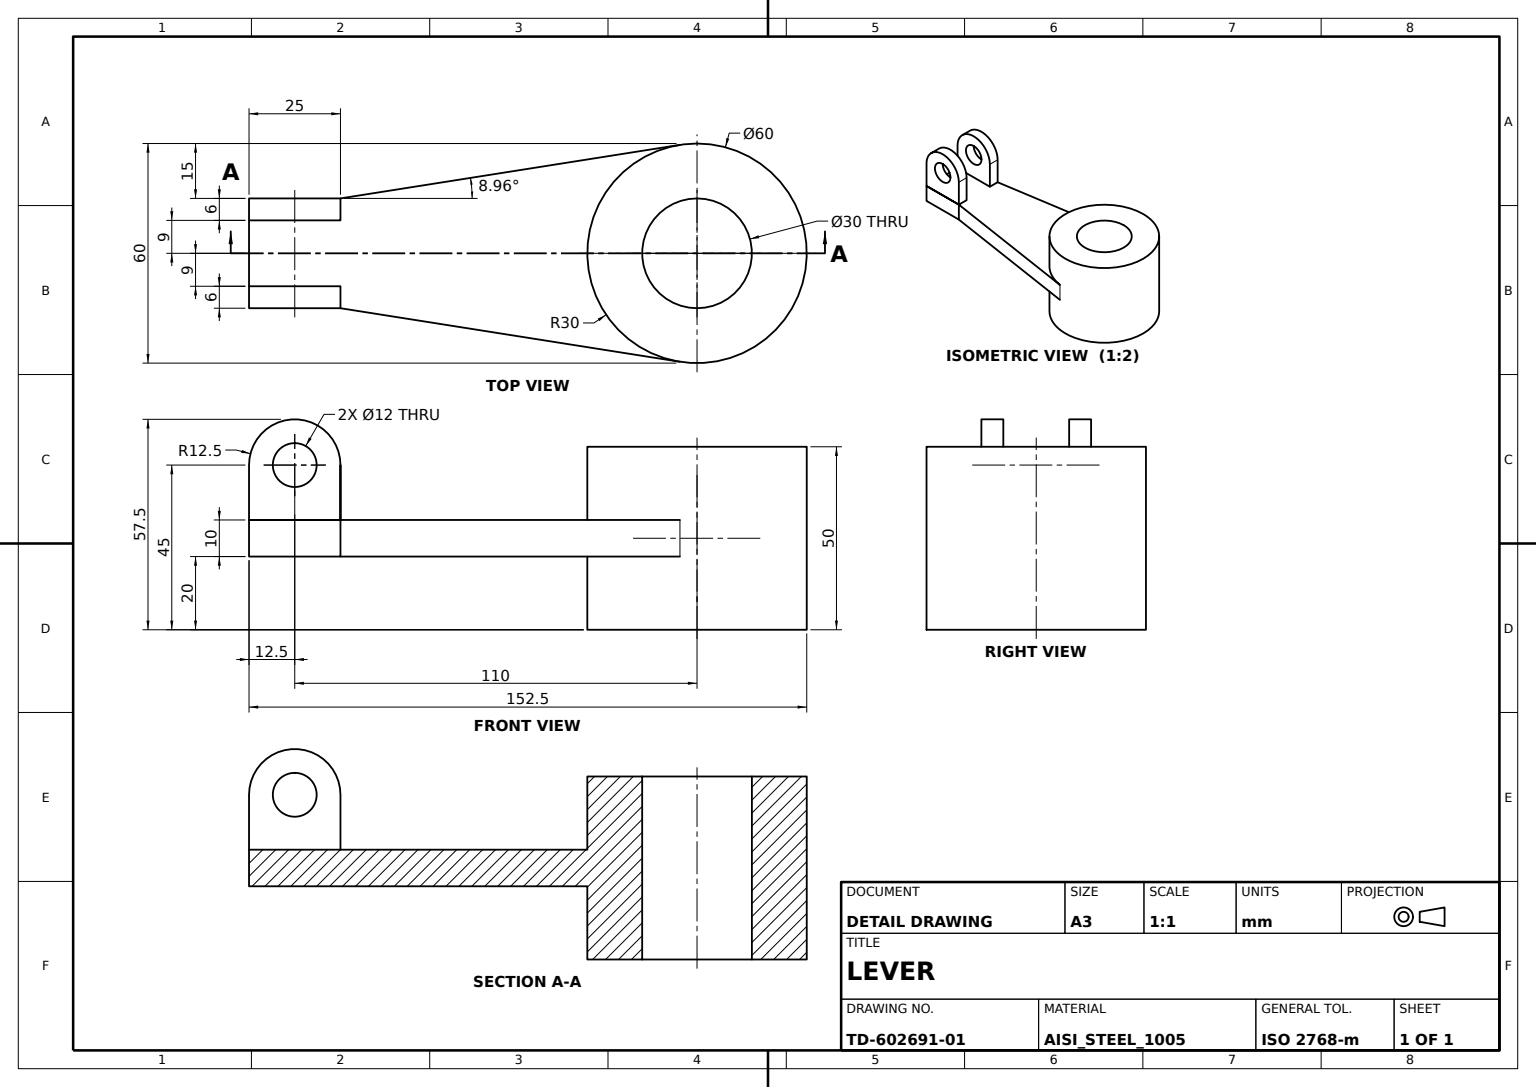
ISO-10303-21;
HEADER;
FILE_DESCRIPTION((''),'2;1');
FILE_NAME('','',(''),(''),'','','');
FILE_SCHEMA(('AUTOMOTIVE_DESIGN'));
ENDSEC;
DATA;
#1=APPLICATION_CONTEXT('');
#2=PRODUCT_CONTEXT('',#1,'mechanical');
#3=PRODUCT('','','',(#2));
#4=PRODUCT_DEFINITION_FORMATION('','',#3);
#5=PRODUCT_DEFINITION_CONTEXT('',#1,'design');
#6=PRODUCT_DEFINITION('','',#4,#5);
#7=PRODUCT_DEFINITION_SHAPE('','',#6);
#8=(LENGTH_UNIT()NAMED_UNIT(*)SI_UNIT(.MILLI.,.METRE.));
#9=(NAMED_UNIT(*)PLANE_ANGLE_UNIT()SI_UNIT($,.RADIAN.));
#10=(NAMED_UNIT(*)SI_UNIT($,.STERADIAN.)SOLID_ANGLE_UNIT());
#11=UNCERTAINTY_MEASURE_WITH_UNIT(LENGTH_MEASURE(0.005),#8,'distance_accuracy_value','');
#12=(GEOMETRIC_REPRESENTATION_CONTEXT(3)GLOBAL_UNCERTAINTY_ASSIGNED_CONTEXT((#11))GLOBAL_UNIT_ASSIGNED_CONTEXT((#8,#9,#10))REPRESENTATION_CONTEXT('',''));
#13=CARTESIAN_POINT('',(-122.5,9.,5.));
#14=VERTEX_POINT('',#13);
#15=CARTESIAN_POINT('',(-122.5,15.,5.));
#16=VERTEX_POINT('',#15);
#17=DIRECTION('',(0.,1.,0.));
#18=VECTOR('',#17,1000.);
#19=LINE('',#13,#18);
#20=EDGE_CURVE('',#14,#16,#19,.T.);
#21=ORIENTED_EDGE('',*,*,#20,.F.);
#22=CARTESIAN_POINT('',(-122.5,9.,20.));
#23=VERTEX_POINT('',#22);
#24=DIRECTION('',(0.,0.,-1.));
#25=VECTOR('',#24,1000.);
#26=LINE('',#22,#25);
#27=EDGE_CURVE('',#23,#14,#26,.T.);
#28=ORIENTED_EDGE('',*,*,#27,.F.);
#29=CARTESIAN_POINT('',(-122.5,15.,20.));
#30=VERTEX_POINT('',#29);
#31=LINE('',#22,#18);
#32=EDGE_CURVE('',#23,#30,#31,.T.);
#33=ORIENTED_EDGE('',*,*,#32,.T.);
#34=LINE('',#29,#25);
#35=EDGE_CURVE('',#30,#16,#34,.T.);
#36=ORIENTED_EDGE('',*,*,#35,.T.);
#37=EDGE_LOOP('',(#21,#28,#33,#36));
#38=FACE_BOUND('',#37,.T.);
#39=DIRECTION('',(1.,0.,0.));
#40=AXIS2_PLACEMENT_3D('',#22,#39,#17);
#41=PLANE('',#40);
#42=ADVANCED_FACE('',(#38),#41,.F.);
#43=CARTESIAN_POINT('',(-110.,9.,26.));
#44=VERTEX_POINT('',#43);
#45=CARTESIAN_POINT('',(-110.,9.,20.));
#46=DIRECTION('',(0.,-1.,0.));
#47=DIRECTION('',(0.,0.,1.));
#48=AXIS2_PLACEMENT_3D('',#45,#46,#47);
#49=CIRCLE('',#48,6.);
#50=EDGE_CURVE('',#44,#44,#49,.T.);
#51=ORIENTED_EDGE('',*,*,#50,.T.);
#52=EDGE_LOOP('',(#51));
#53=FACE_BOUND('',#52,.T.);
#54=CARTESIAN_POINT('',(-110.,15.,26.));
#55=VERTEX_POINT('',#54);
#56=CARTESIAN_POINT('',(-110.,15.,20.));
#57=AXIS2_PLACEMENT_3D('',#56,#46,#47);
#58=CIRCLE('',#57,6.);
#59=EDGE_CURVE('',#55,#55,#58,.T.);
#60=ORIENTED_EDGE('',*,*,#59,.F.);
#61=EDGE_LOOP('',(#60));
#62=FACE_BOUND('',#61,.T.);
#63=DIRECTION('',(-1.,0.,0.));
#64=AXIS2_PLACEMENT_3D('',#45,#17,#63);
#65=CYLINDRICAL_SURFACE('',#64,6.);
#66=ADVANCED_FACE('',(#53,#62),#65,.F.);
#67=CARTESIAN_POINT('',(-97.5,9.,5.));
#68=VERTEX_POINT('',#67);
#69=CARTESIAN_POINT('',(-97.5,15.,5.));
#70=VERTEX_POINT('',#69);
#71=LINE('',#67,#18);
#72=EDGE_CURVE('',#68,#70,#71,.T.);
#73=ORIENTED_EDGE('',*,*,#72,.F.);
#74=VECTOR('',#39,1000.);
#75=LINE('',#13,#74);
#76=EDGE_CURVE('',#14,#68,#75,.T.);
#77=ORIENTED_EDGE('',*,*,#76,.F.);
#78=ORIENTED_EDGE('',*,*,#20,.T.);
#79=LINE('',#15,#74);
#80=EDGE_CURVE('',#16,#70,#79,.T.);
#81=ORIENTED_EDGE('',*,*,#80,.T.);
#82=EDGE_LOOP('',(#73,#77,#78,#81));
#83=FACE_BOUND('',#82,.T.);
#84=AXIS2_PLACEMENT_3D('',#13,#47,#39);
#85=PLANE('',#84);
#86=ADVANCED_FACE('',(#83),#85,.F.);
#87=ORIENTED_EDGE('',*,*,#32,.F.);
#88=CARTESIAN_POINT('',(-97.5,9.,20.));
#89=VERTEX_POINT('',#88);
#90=CIRCLE('',#48,12.5);
#91=EDGE_CURVE('',#89,#23,#90,.T.);
#92=ORIENTED_EDGE('',*,*,#91,.F.);
#93=CARTESIAN_POINT('',(-97.5,15.,20.));
#94=VERTEX_POINT('',#93);
#95=LINE('',#88,#18);
#96=EDGE_CURVE('',#89,#94,#95,.T.);
#97=ORIENTED_EDGE('',*,*,#96,.T.);
#98=CIRCLE('',#57,12.5);
#99=EDGE_CURVE('',#94,#30,#98,.T.);
#100=ORIENTED_EDGE('',*,*,#99,.T.);
#101=EDGE_LOOP('',(#87,#92,#97,#100));
#102=FACE_BOUND('',#101,.T.);
#103=CYLINDRICAL_SURFACE('',#64,12.5);
#104=ADVANCED_FACE('',(#102),#103,.T.);
#105=ORIENTED_EDGE('',*,*,#96,.F.);
#106=VECTOR('',#47,1000.);
#107=LINE('',#67,#106);
#108=EDGE_CURVE('',#68,#89,#107,.T.);
#109=ORIENTED_EDGE('',*,*,#108,.F.);
#110=ORIENTED_EDGE('',*,*,#72,.T.);
#111=LINE('',#69,#106);
#112=EDGE_CURVE('',#70,#94,#111,.T.);
#113=ORIENTED_EDGE('',*,*,#112,.T.);
#114=EDGE_LOOP('',(#105,#109,#110,#113));
#115=FACE_BOUND('',#114,.T.);
#116=AXIS2_PLACEMENT_3D('',#67,#63,#46);
#117=PLANE('',#116);
#118=ADVANCED_FACE('',(#115),#117,.F.);
#119=ORIENTED_EDGE('',*,*,#59,.T.);
#120=EDGE_LOOP('',(#119));
#121=FACE_BOUND('',#120,.T.);
#122=ORIENTED_EDGE('',*,*,#80,.F.);
#123=ORIENTED_EDGE('',*,*,#35,.F.);
#124=ORIENTED_EDGE('',*,*,#99,.F.);
#125=ORIENTED_EDGE('',*,*,#112,.F.);
#126=EDGE_LOOP('',(#122,#123,#124,#125));
#127=FACE_BOUND('',#126,.T.);
#128=AXIS2_PLACEMENT_3D('',#56,#46,#39);
#129=PLANE('',#128);
#130=ADVANCED_FACE('',(#121,#127),#129,.F.);
#131=ORIENTED_EDGE('',*,*,#108,.T.);
#132=ORIENTED_EDGE('',*,*,#91,.T.);
#133=ORIENTED_EDGE('',*,*,#27,.T.);
#134=ORIENTED_EDGE('',*,*,#76,.T.);
#135=EDGE_LOOP('',(#131,#132,#133,#134));
#136=FACE_BOUND('',#135,.T.);
#137=ORIENTED_EDGE('',*,*,#50,.F.);
#138=EDGE_LOOP('',(#137));
#139=FACE_BOUND('',#138,.T.);
#140=AXIS2_PLACEMENT_3D('',#45,#46,#39);
#141=PLANE('',#140);
#142=ADVANCED_FACE('',(#136,#139),#141,.T.);
#143=CLOSED_SHELL('',(#42,#66,#86,#104,#118,#130,#142));
#144=MANIFOLD_SOLID_BREP('',#143);
#145=CARTESIAN_POINT('',(-122.5,-9.,5.));
#146=VERTEX_POINT('',#145);
#147=CARTESIAN_POINT('',(-97.5,-9.,5.));
#148=VERTEX_POINT('',#147);
#149=LINE('',#145,#74);
#150=EDGE_CURVE('',#146,#148,#149,.T.);
#151=ORIENTED_EDGE('',*,*,#150,.T.);
#152=CARTESIAN_POINT('',(-97.5,-15.,5.));
#153=VERTEX_POINT('',#152);
#154=VECTOR('',#46,1000.);
#155=LINE('',#147,#154);
#156=EDGE_CURVE('',#148,#153,#155,.T.);
#157=ORIENTED_EDGE('',*,*,#156,.T.);
#158=CARTESIAN_POINT('',(-122.5,-15.,5.));
#159=VERTEX_POINT('',#158);
#160=LINE('',#158,#74);
#161=EDGE_CURVE('',#159,#153,#160,.T.);
#162=ORIENTED_EDGE('',*,*,#161,.F.);
#163=LINE('',#145,#154);
#164=EDGE_CURVE('',#146,#159,#163,.T.);
#165=ORIENTED_EDGE('',*,*,#164,.F.);
#166=EDGE_LOOP('',(#151,#157,#162,#165));
#167=FACE_BOUND('',#166,.T.);
#168=AXIS2_PLACEMENT_3D('',#145,#24,#63);
#169=PLANE('',#168);
#170=ADVANCED_FACE('',(#167),#169,.T.);
#171=CARTESIAN_POINT('',(-97.5,-15.,20.));
#172=VERTEX_POINT('',#171);
#173=CARTESIAN_POINT('',(-122.5,-15.,20.));
#174=VERTEX_POINT('',#173);
#175=CARTESIAN_POINT('',(-110.,-15.,20.));
#176=AXIS2_PLACEMENT_3D('',#175,#46,#47);
#177=CIRCLE('',#176,12.5);
#178=EDGE_CURVE('',#172,#174,#177,.T.);
#179=ORIENTED_EDGE('',*,*,#178,.F.);
#180=CARTESIAN_POINT('',(-97.5,-9.,20.));
#181=VERTEX_POINT('',#180);
#182=LINE('',#180,#154);
#183=EDGE_CURVE('',#181,#172,#182,.T.);
#184=ORIENTED_EDGE('',*,*,#183,.F.);
#185=CARTESIAN_POINT('',(-122.5,-9.,20.));
#186=VERTEX_POINT('',#185);
#187=CARTESIAN_POINT('',(-110.,-9.,20.));
#188=AXIS2_PLACEMENT_3D('',#187,#46,#47);
#189=CIRCLE('',#188,12.5);
#190=EDGE_CURVE('',#181,#186,#189,.T.);
#191=ORIENTED_EDGE('',*,*,#190,.T.);
#192=LINE('',#185,#154);
#193=EDGE_CURVE('',#186,#174,#192,.T.);
#194=ORIENTED_EDGE('',*,*,#193,.T.);
#195=EDGE_LOOP('',(#179,#184,#191,#194));
#196=FACE_BOUND('',#195,.T.);
#197=AXIS2_PLACEMENT_3D('',#187,#46,#39);
#198=CYLINDRICAL_SURFACE('',#197,12.5);
#199=ADVANCED_FACE('',(#196),#198,.T.);
#200=CARTESIAN_POINT('',(-110.,-9.,26.));
#201=VERTEX_POINT('',#200);
#202=CIRCLE('',#188,6.);
#203=EDGE_CURVE('',#201,#201,#202,.T.);
#204=ORIENTED_EDGE('',*,*,#203,.F.);
#205=EDGE_LOOP('',(#204));
#206=FACE_BOUND('',#205,.T.);
#207=CARTESIAN_POINT('',(-110.,-15.,26.));
#208=VERTEX_POINT('',#207);
#209=CIRCLE('',#176,6.);
#210=EDGE_CURVE('',#208,#208,#209,.T.);
#211=ORIENTED_EDGE('',*,*,#210,.T.);
#212=EDGE_LOOP('',(#211));
#213=FACE_BOUND('',#212,.T.);
#214=CYLINDRICAL_SURFACE('',#197,6.);
#215=ADVANCED_FACE('',(#206,#213),#214,.F.);
#216=ORIENTED_EDGE('',*,*,#203,.T.);
#217=EDGE_LOOP('',(#216));
#218=FACE_BOUND('',#217,.T.);
#219=ORIENTED_EDGE('',*,*,#190,.F.);
#220=LINE('',#147,#106);
#221=EDGE_CURVE('',#148,#181,#220,.T.);
#222=ORIENTED_EDGE('',*,*,#221,.F.);
#223=ORIENTED_EDGE('',*,*,#150,.F.);
#224=LINE('',#185,#25);
#225=EDGE_CURVE('',#186,#146,#224,.T.);
#226=ORIENTED_EDGE('',*,*,#225,.F.);
#227=EDGE_LOOP('',(#219,#222,#223,#226));
#228=FACE_BOUND('',#227,.T.);
#229=PLANE('',#197);
#230=ADVANCED_FACE('',(#218,#228),#229,.F.);
#231=ORIENTED_EDGE('',*,*,#164,.T.);
#232=LINE('',#173,#25);
#233=EDGE_CURVE('',#174,#159,#232,.T.);
#234=ORIENTED_EDGE('',*,*,#233,.F.);
#235=ORIENTED_EDGE('',*,*,#193,.F.);
#236=ORIENTED_EDGE('',*,*,#225,.T.);
#237=EDGE_LOOP('',(#231,#234,#235,#236));
#238=FACE_BOUND('',#237,.T.);
#239=AXIS2_PLACEMENT_3D('',#185,#63,#46);
#240=PLANE('',#239);
#241=ADVANCED_FACE('',(#238),#240,.T.);
#242=LINE('',#152,#106);
#243=EDGE_CURVE('',#153,#172,#242,.T.);
#244=ORIENTED_EDGE('',*,*,#243,.F.);
#245=ORIENTED_EDGE('',*,*,#156,.F.);
#246=ORIENTED_EDGE('',*,*,#221,.T.);
#247=ORIENTED_EDGE('',*,*,#183,.T.);
#248=EDGE_LOOP('',(#244,#245,#246,#247));
#249=FACE_BOUND('',#248,.T.);
#250=AXIS2_PLACEMENT_3D('',#147,#39,#17);
#251=PLANE('',#250);
#252=ADVANCED_FACE('',(#249),#251,.T.);
#253=ORIENTED_EDGE('',*,*,#210,.F.);
#254=EDGE_LOOP('',(#253));
#255=FACE_BOUND('',#254,.T.);
#256=ORIENTED_EDGE('',*,*,#161,.T.);
#257=ORIENTED_EDGE('',*,*,#243,.T.);
#258=ORIENTED_EDGE('',*,*,#178,.T.);
#259=ORIENTED_EDGE('',*,*,#233,.T.);
#260=EDGE_LOOP('',(#256,#257,#258,#259));
#261=FACE_BOUND('',#260,.T.);
#262=AXIS2_PLACEMENT_3D('',#175,#46,#39);
#263=PLANE('',#262);
#264=ADVANCED_FACE('',(#255,#261),#263,.T.);
#265=CLOSED_SHELL('',(#170,#199,#215,#230,#241,#252,#264));
#266=MANIFOLD_SOLID_BREP('',#265);
#267=VERTEX_POINT('',#15);
#268=VERTEX_POINT('',#158);
#269=LINE('',#15,#154);
#270=EDGE_CURVE('',#267,#268,#269,.T.);
#271=ORIENTED_EDGE('',*,*,#270,.F.);
#272=CARTESIAN_POINT('',(-122.5,15.,-5.));
#273=VERTEX_POINT('',#272);
#274=LINE('',#15,#25);
#275=EDGE_CURVE('',#267,#273,#274,.T.);
#276=ORIENTED_EDGE('',*,*,#275,.T.);
#277=CARTESIAN_POINT('',(-122.5,-15.,-5.));
#278=VERTEX_POINT('',#277);
#279=LINE('',#272,#154);
#280=EDGE_CURVE('',#273,#278,#279,.T.);
#281=ORIENTED_EDGE('',*,*,#280,.T.);
#282=LINE('',#158,#25);
#283=EDGE_CURVE('',#268,#278,#282,.T.);
#284=ORIENTED_EDGE('',*,*,#283,.F.);
#285=EDGE_LOOP('',(#271,#276,#281,#284));
#286=FACE_BOUND('',#285,.T.);
#287=AXIS2_PLACEMENT_3D('',#15,#39,#24);
#288=PLANE('',#287);
#289=ADVANCED_FACE('',(#286),#288,.F.);
#290=ORIENTED_EDGE('',*,*,#270,.T.);
#291=VERTEX_POINT('',#152);
#292=EDGE_CURVE('',#268,#291,#160,.T.);
#293=ORIENTED_EDGE('',*,*,#292,.T.);
#294=CARTESIAN_POINT('',(-4.671689,-29.634023,5.));
#295=VERTEX_POINT('',#294);
#296=DIRECTION('',(0.987800769,-0.155722959,0.));
#297=VECTOR('',#296,1000.);
#298=LINE('',#152,#297);
#299=EDGE_CURVE('',#291,#295,#298,.T.);
#300=ORIENTED_EDGE('',*,*,#299,.T.);
#301=CARTESIAN_POINT('',(-4.671689,29.634023,5.));
#302=VERTEX_POINT('',#301);
#303=CARTESIAN_POINT('',(0.,0.,5.));
#304=AXIS2_PLACEMENT_3D('',#303,#24,#17);
#305=CIRCLE('',#304,30.);
#306=EDGE_CURVE('',#295,#302,#305,.T.);
#307=ORIENTED_EDGE('',*,*,#306,.T.);
#308=VERTEX_POINT('',#69);
#309=DIRECTION('',(-0.987800769,-0.155722959,0.));
#310=VECTOR('',#309,1000.);
#311=LINE('',#301,#310);
#312=EDGE_CURVE('',#302,#308,#311,.T.);
#313=ORIENTED_EDGE('',*,*,#312,.T.);
#314=VECTOR('',#63,1000.);
#315=LINE('',#69,#314);
#316=EDGE_CURVE('',#308,#267,#315,.T.);
#317=ORIENTED_EDGE('',*,*,#316,.T.);
#318=EDGE_LOOP('',(#290,#293,#300,#307,#313,#317));
#319=FACE_BOUND('',#318,.T.);
#320=AXIS2_PLACEMENT_3D('',#303,#24,#63);
#321=PLANE('',#320);
#322=ADVANCED_FACE('',(#319),#321,.F.);
#323=ORIENTED_EDGE('',*,*,#316,.F.);
#324=CARTESIAN_POINT('',(-97.5,15.,-5.));
#325=VERTEX_POINT('',#324);
#326=LINE('',#69,#25);
#327=EDGE_CURVE('',#308,#325,#326,.T.);
#328=ORIENTED_EDGE('',*,*,#327,.T.);
#329=LINE('',#324,#314);
#330=EDGE_CURVE('',#325,#273,#329,.T.);
#331=ORIENTED_EDGE('',*,*,#330,.T.);
#332=ORIENTED_EDGE('',*,*,#275,.F.);
#333=EDGE_LOOP('',(#323,#328,#331,#332));
#334=FACE_BOUND('',#333,.T.);
#335=AXIS2_PLACEMENT_3D('',#69,#46,#39);
#336=PLANE('',#335);
#337=ADVANCED_FACE('',(#334),#336,.F.);
#338=CARTESIAN_POINT('',(-97.5,-15.,-5.));
#339=VERTEX_POINT('',#338);
#340=LINE('',#152,#25);
#341=EDGE_CURVE('',#291,#339,#340,.T.);
#342=ORIENTED_EDGE('',*,*,#341,.F.);
#343=ORIENTED_EDGE('',*,*,#292,.F.);
#344=ORIENTED_EDGE('',*,*,#283,.T.);
#345=LINE('',#277,#74);
#346=EDGE_CURVE('',#278,#339,#345,.T.);
#347=ORIENTED_EDGE('',*,*,#346,.T.);
#348=EDGE_LOOP('',(#342,#343,#344,#347));
#349=FACE_BOUND('',#348,.T.);
#350=AXIS2_PLACEMENT_3D('',#158,#17,#63);
#351=PLANE('',#350);
#352=ADVANCED_FACE('',(#349),#351,.F.);
#353=CARTESIAN_POINT('',(0.,15.,-25.));
#354=VERTEX_POINT('',#353);
#355=CARTESIAN_POINT('',(0.,0.,-25.));
#356=AXIS2_PLACEMENT_3D('',#355,#47,#17);
#357=CIRCLE('',#356,15.);
#358=EDGE_CURVE('',#354,#354,#357,.T.);
#359=ORIENTED_EDGE('',*,*,#358,.T.);
#360=EDGE_LOOP('',(#359));
#361=FACE_BOUND('',#360,.T.);
#362=CARTESIAN_POINT('',(0.,30.,-25.));
#363=VERTEX_POINT('',#362);
#364=CIRCLE('',#356,30.);
#365=EDGE_CURVE('',#363,#363,#364,.T.);
#366=ORIENTED_EDGE('',*,*,#365,.F.);
#367=EDGE_LOOP('',(#366));
#368=FACE_BOUND('',#367,.T.);
#369=AXIS2_PLACEMENT_3D('',#355,#47,#39);
#370=PLANE('',#369);
#371=ADVANCED_FACE('',(#361,#368),#370,.F.);
#372=CARTESIAN_POINT('',(-4.671689,29.634023,-5.));
#373=VERTEX_POINT('',#372);
#374=LINE('',#372,#310);
#375=EDGE_CURVE('',#373,#325,#374,.T.);
#376=ORIENTED_EDGE('',*,*,#375,.F.);
#377=CARTESIAN_POINT('',(-4.671689,-29.634023,-5.));
#378=VERTEX_POINT('',#377);
#379=CARTESIAN_POINT('',(0.,0.,-5.));
#380=AXIS2_PLACEMENT_3D('',#379,#24,#17);
#381=CIRCLE('',#380,30.);
#382=EDGE_CURVE('',#378,#373,#381,.T.);
#383=ORIENTED_EDGE('',*,*,#382,.F.);
#384=LINE('',#338,#297);
#385=EDGE_CURVE('',#339,#378,#384,.T.);
#386=ORIENTED_EDGE('',*,*,#385,.F.);
#387=ORIENTED_EDGE('',*,*,#346,.F.);
#388=ORIENTED_EDGE('',*,*,#280,.F.);
#389=ORIENTED_EDGE('',*,*,#330,.F.);
#390=EDGE_LOOP('',(#376,#383,#386,#387,#388,#389));
#391=FACE_BOUND('',#390,.T.);
#392=AXIS2_PLACEMENT_3D('',#379,#24,#63);
#393=PLANE('',#392);
#394=ADVANCED_FACE('',(#391),#393,.T.);
#395=ORIENTED_EDGE('',*,*,#365,.T.);
#396=EDGE_LOOP('',(#395));
#397=FACE_BOUND('',#396,.T.);
#398=CARTESIAN_POINT('',(0.,30.,25.));
#399=VERTEX_POINT('',#398);
#400=CARTESIAN_POINT('',(0.,0.,25.));
#401=AXIS2_PLACEMENT_3D('',#400,#47,#17);
#402=CIRCLE('',#401,30.);
#403=EDGE_CURVE('',#399,#399,#402,.T.);
#404=ORIENTED_EDGE('',*,*,#403,.F.);
#405=EDGE_LOOP('',(#404));
#406=FACE_BOUND('',#405,.T.);
#407=ORIENTED_EDGE('',*,*,#382,.T.);
#408=LINE('',#301,#25);
#409=EDGE_CURVE('',#302,#373,#408,.T.);
#410=ORIENTED_EDGE('',*,*,#409,.F.);
#411=ORIENTED_EDGE('',*,*,#306,.F.);
#412=LINE('',#294,#25);
#413=EDGE_CURVE('',#295,#378,#412,.T.);
#414=ORIENTED_EDGE('',*,*,#413,.T.);
#415=EDGE_LOOP('',(#407,#410,#411,#414));
#416=FACE_BOUND('',#415,.T.);
#417=AXIS2_PLACEMENT_3D('',#400,#24,#63);
#418=CYLINDRICAL_SURFACE('',#417,30.);
#419=ADVANCED_FACE('',(#397,#406,#416),#418,.T.);
#420=ORIENTED_EDGE('',*,*,#403,.T.);
#421=EDGE_LOOP('',(#420));
#422=FACE_BOUND('',#421,.T.);
#423=CARTESIAN_POINT('',(0.,15.,25.));
#424=VERTEX_POINT('',#423);
#425=CIRCLE('',#401,15.);
#426=EDGE_CURVE('',#424,#424,#425,.T.);
#427=ORIENTED_EDGE('',*,*,#426,.F.);
#428=EDGE_LOOP('',(#427));
#429=FACE_BOUND('',#428,.T.);
#430=AXIS2_PLACEMENT_3D('',#400,#47,#39);
#431=PLANE('',#430);
#432=ADVANCED_FACE('',(#422,#429),#431,.T.);
#433=ORIENTED_EDGE('',*,*,#375,.T.);
#434=ORIENTED_EDGE('',*,*,#327,.F.);
#435=ORIENTED_EDGE('',*,*,#312,.F.);
#436=ORIENTED_EDGE('',*,*,#409,.T.);
#437=EDGE_LOOP('',(#433,#434,#435,#436));
#438=FACE_BOUND('',#437,.T.);
#439=DIRECTION('',(0.155722959,-0.987800769,0.));
#440=DIRECTION('',(0.987800769,0.155722959,0.));
#441=AXIS2_PLACEMENT_3D('',#301,#439,#440);
#442=PLANE('',#441);
#443=ADVANCED_FACE('',(#438),#442,.F.);
#444=ORIENTED_EDGE('',*,*,#385,.T.);
#445=ORIENTED_EDGE('',*,*,#413,.F.);
#446=ORIENTED_EDGE('',*,*,#299,.F.);
#447=ORIENTED_EDGE('',*,*,#341,.T.);
#448=EDGE_LOOP('',(#444,#445,#446,#447));
#449=FACE_BOUND('',#448,.T.);
#450=DIRECTION('',(0.155722959,0.987800769,0.));
#451=DIRECTION('',(-0.987800769,0.155722959,0.));
#452=AXIS2_PLACEMENT_3D('',#152,#450,#451);
#453=PLANE('',#452);
#454=ADVANCED_FACE('',(#449),#453,.F.);
#455=ORIENTED_EDGE('',*,*,#426,.T.);
#456=EDGE_LOOP('',(#455));
#457=FACE_BOUND('',#456,.T.);
#458=ORIENTED_EDGE('',*,*,#358,.F.);
#459=EDGE_LOOP('',(#458));
#460=FACE_BOUND('',#459,.T.);
#461=CYLINDRICAL_SURFACE('',#417,15.);
#462=ADVANCED_FACE('',(#457,#460),#461,.F.);
#463=CLOSED_SHELL('',(#289,#322,#337,#352,#371,#394,#419,#432,#443,#454,#462));
#464=MANIFOLD_SOLID_BREP('',#463);
#465=ADVANCED_BREP_SHAPE_REPRESENTATION('',(#144,#266,#464),#12);
#466=SHAPE_DEFINITION_REPRESENTATION(#7,#465);
ENDSEC;
END-ISO-10303-21;
